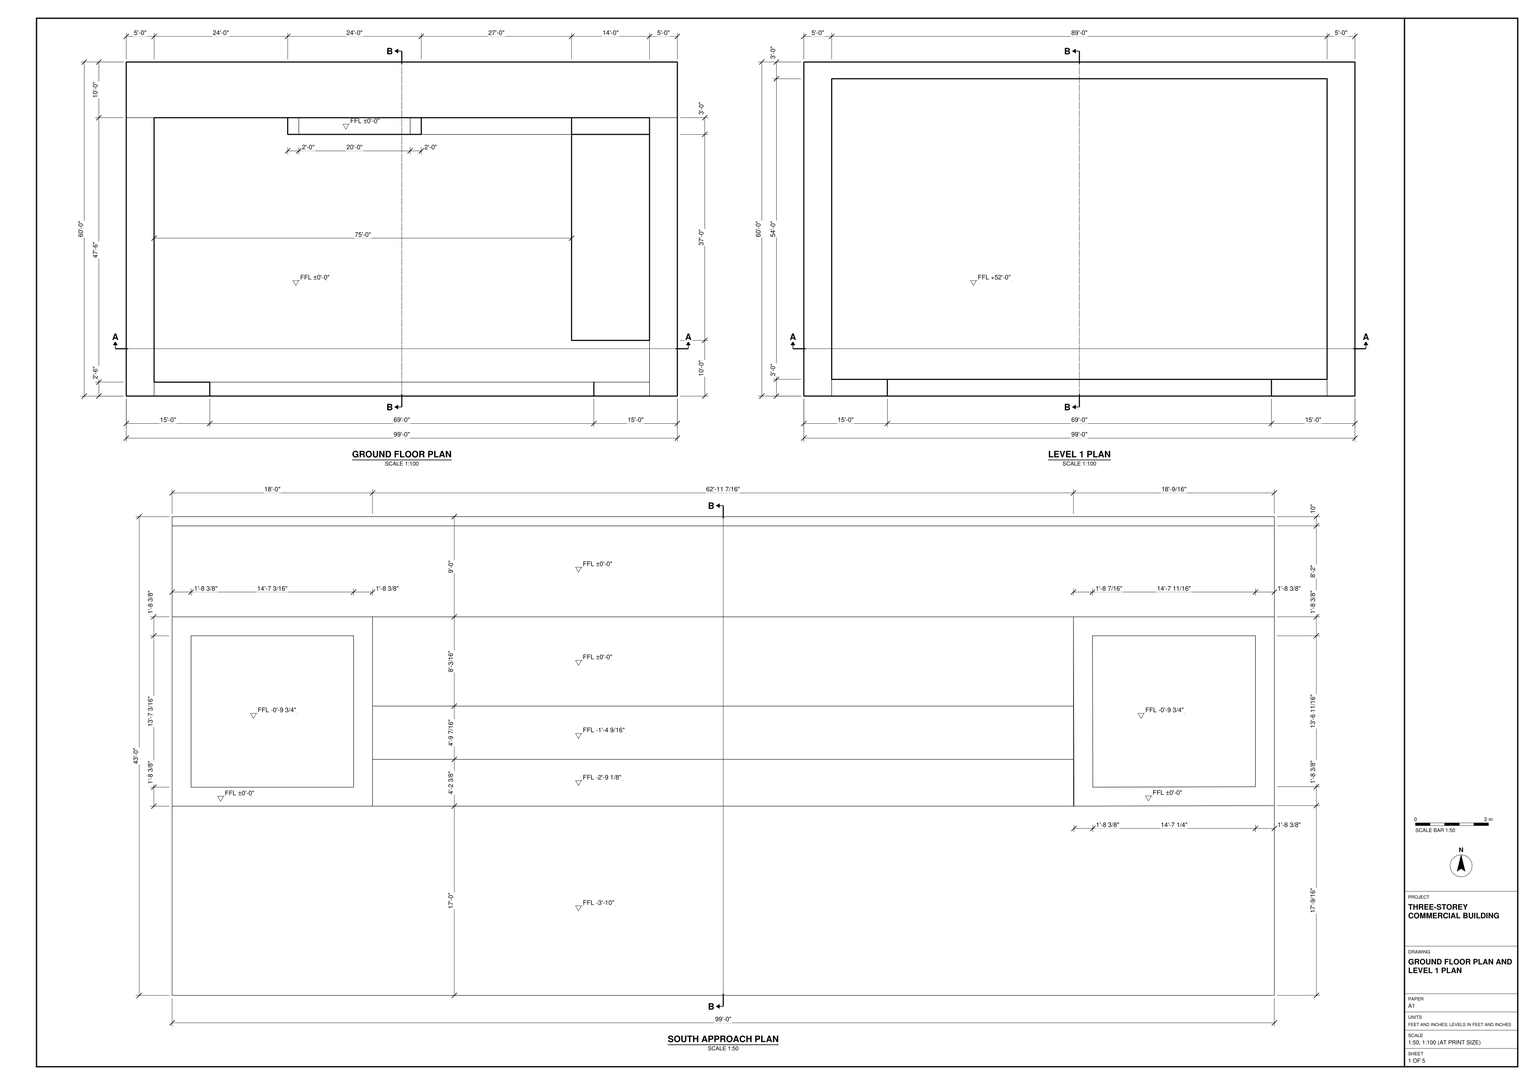
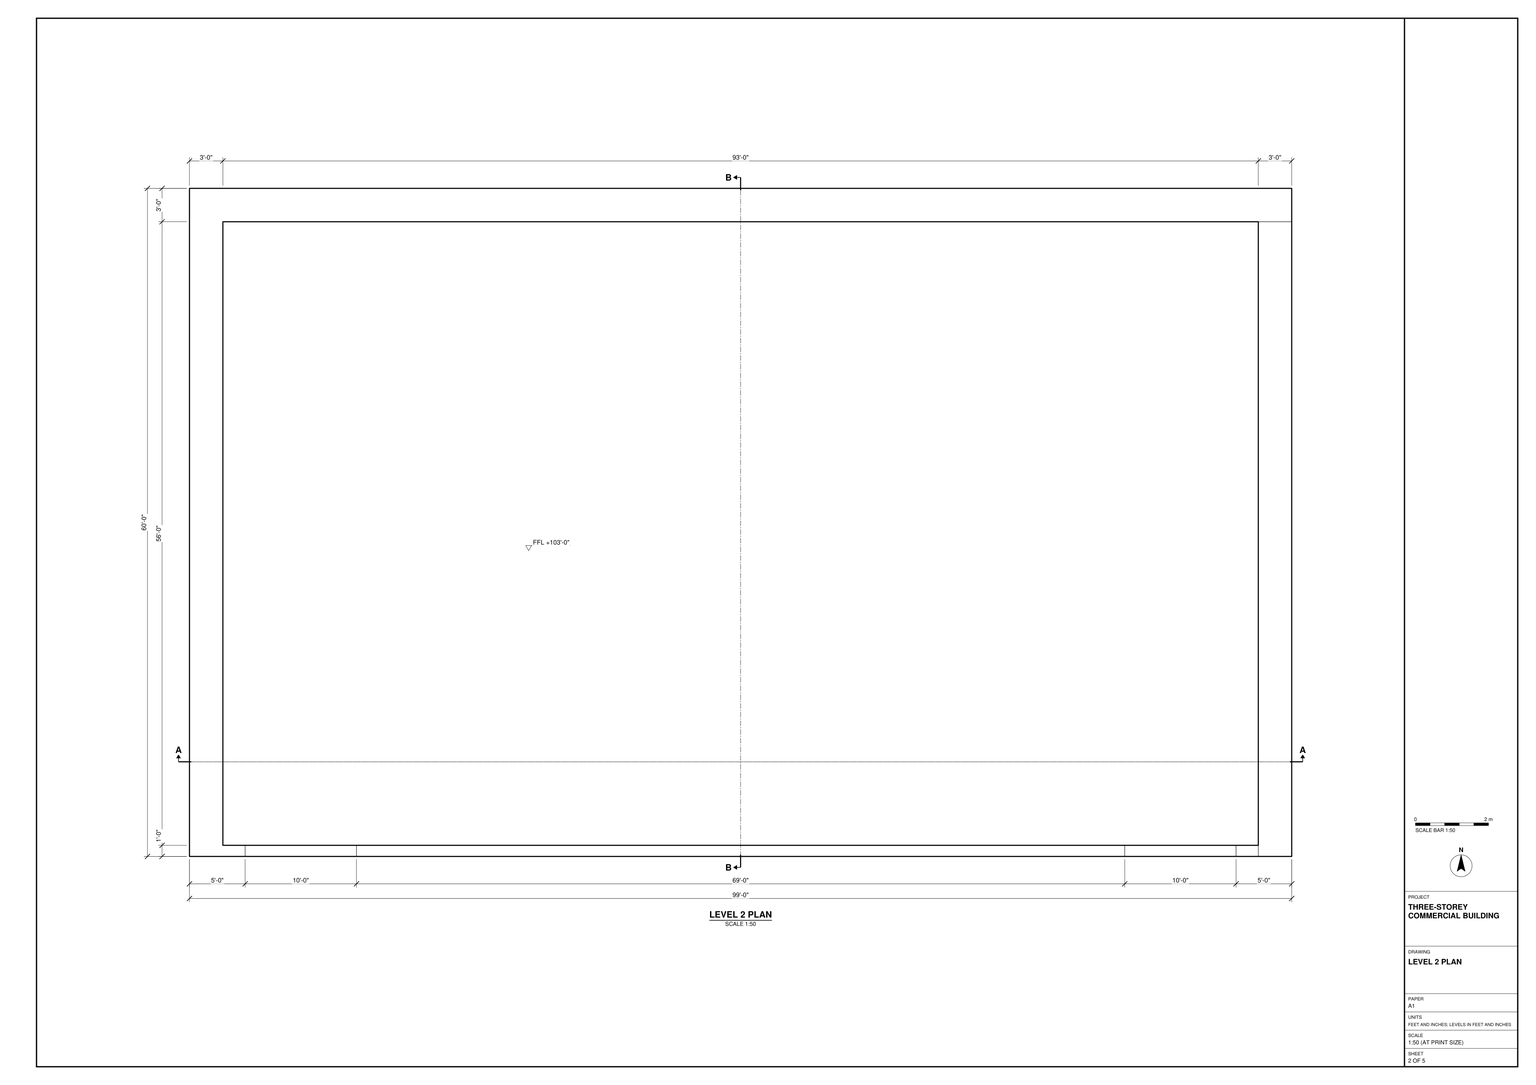
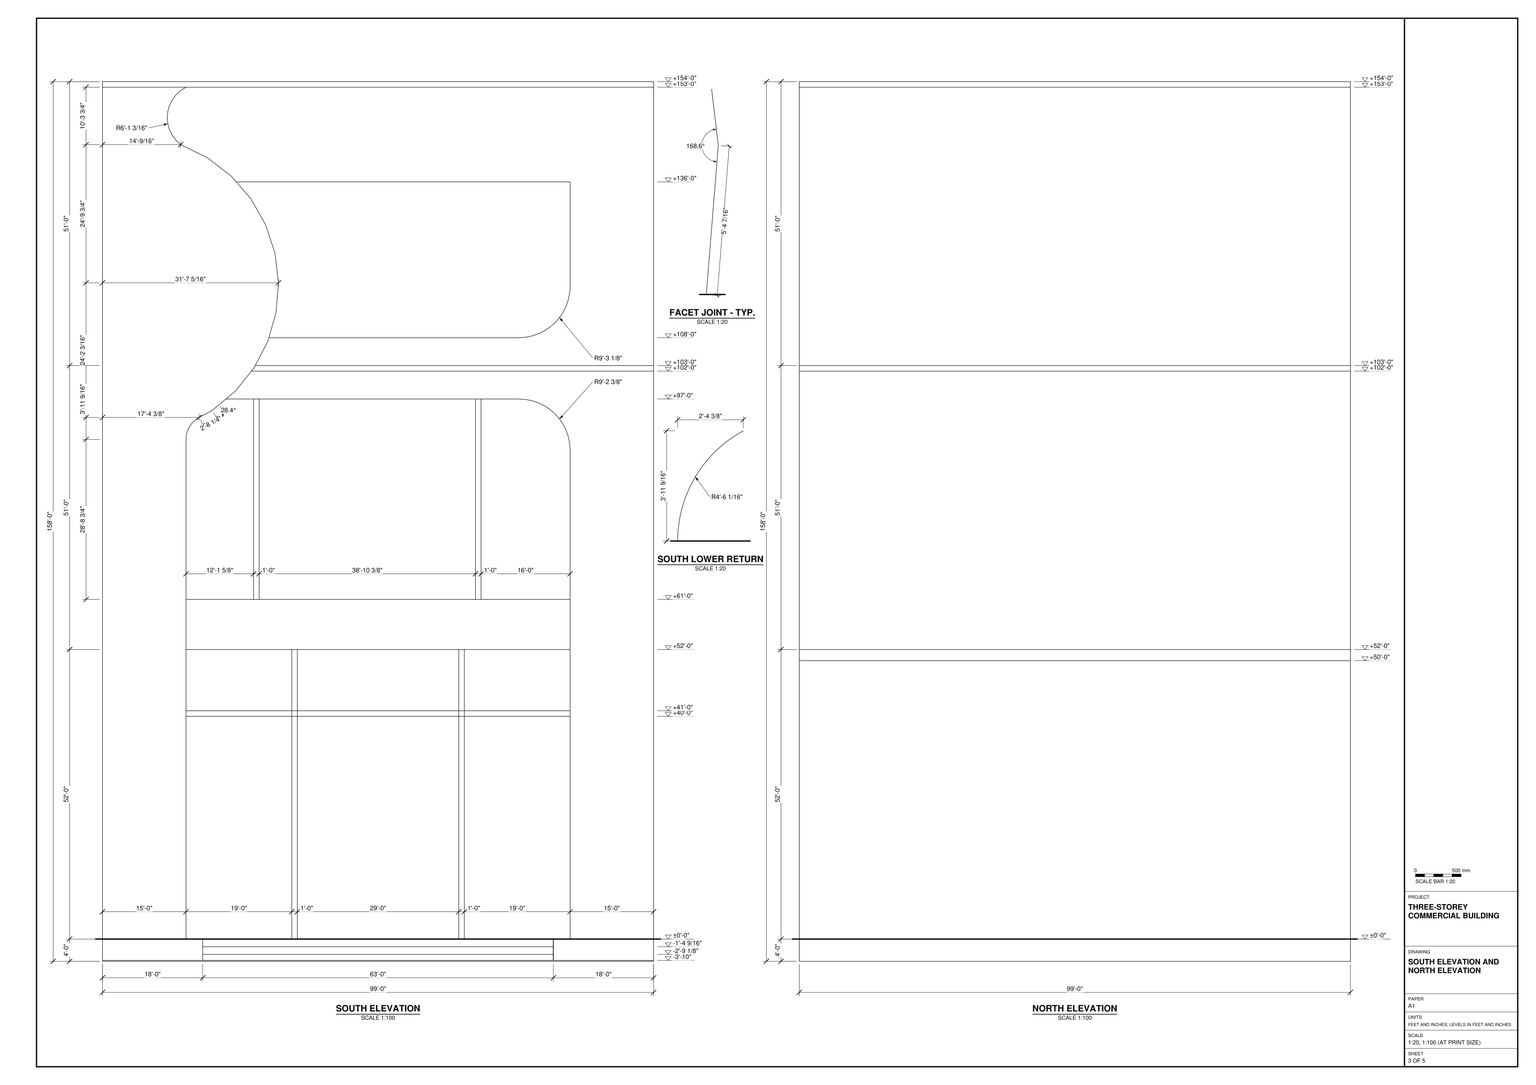
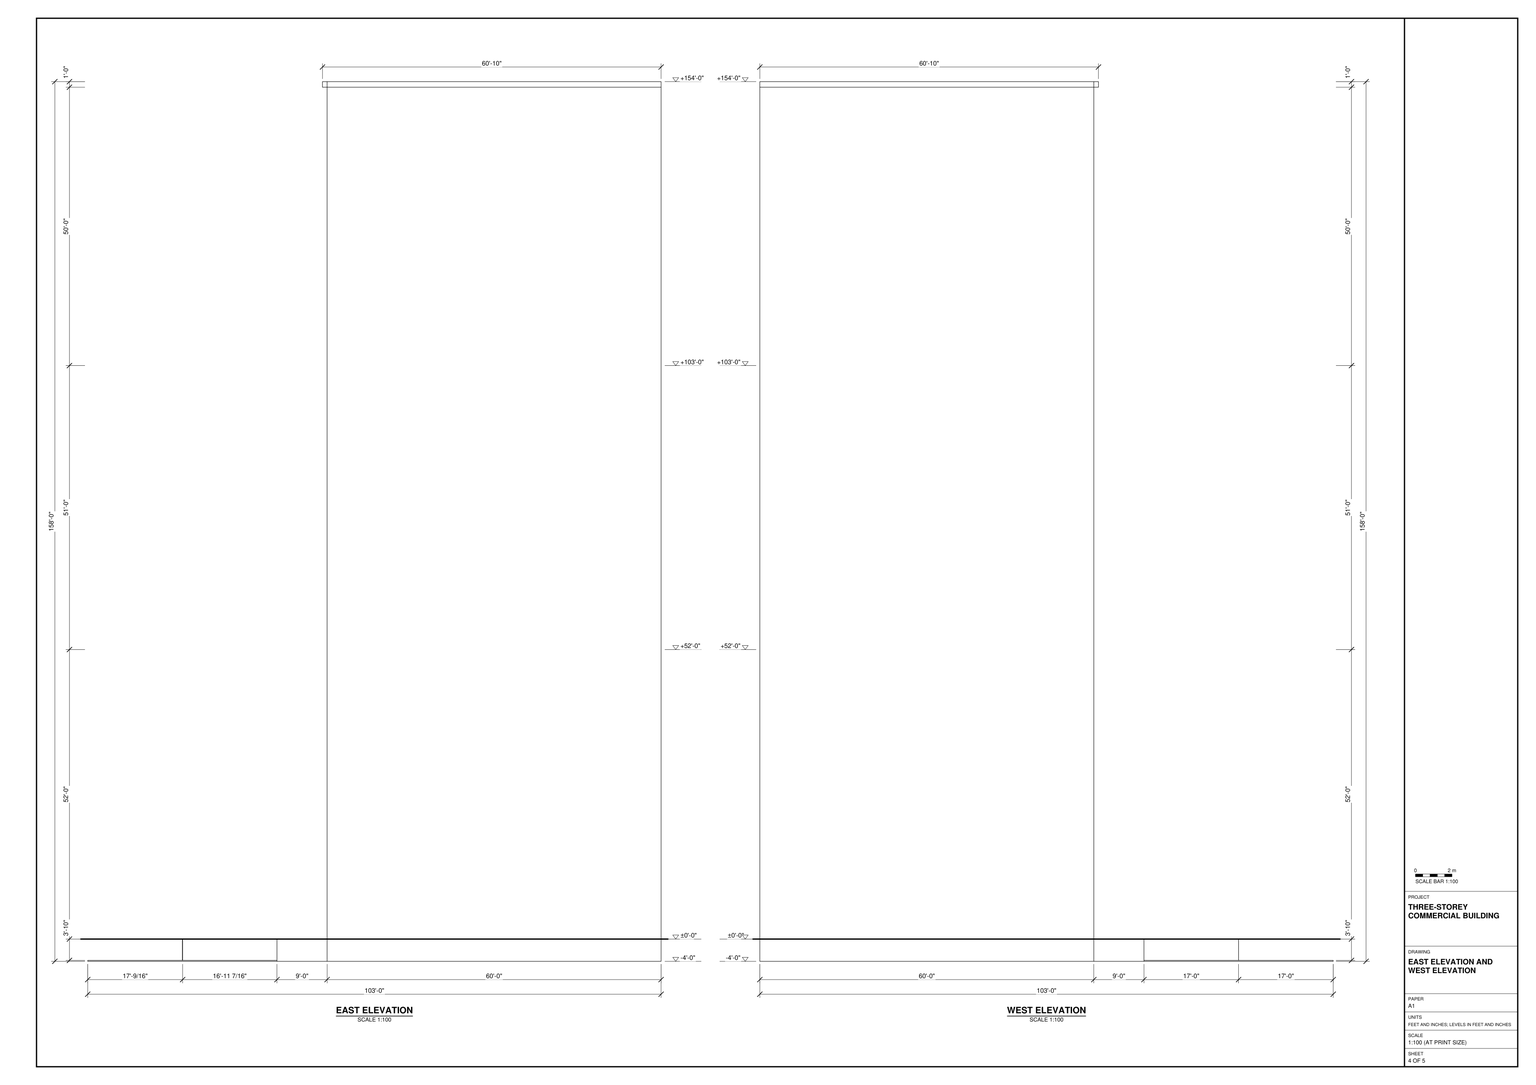
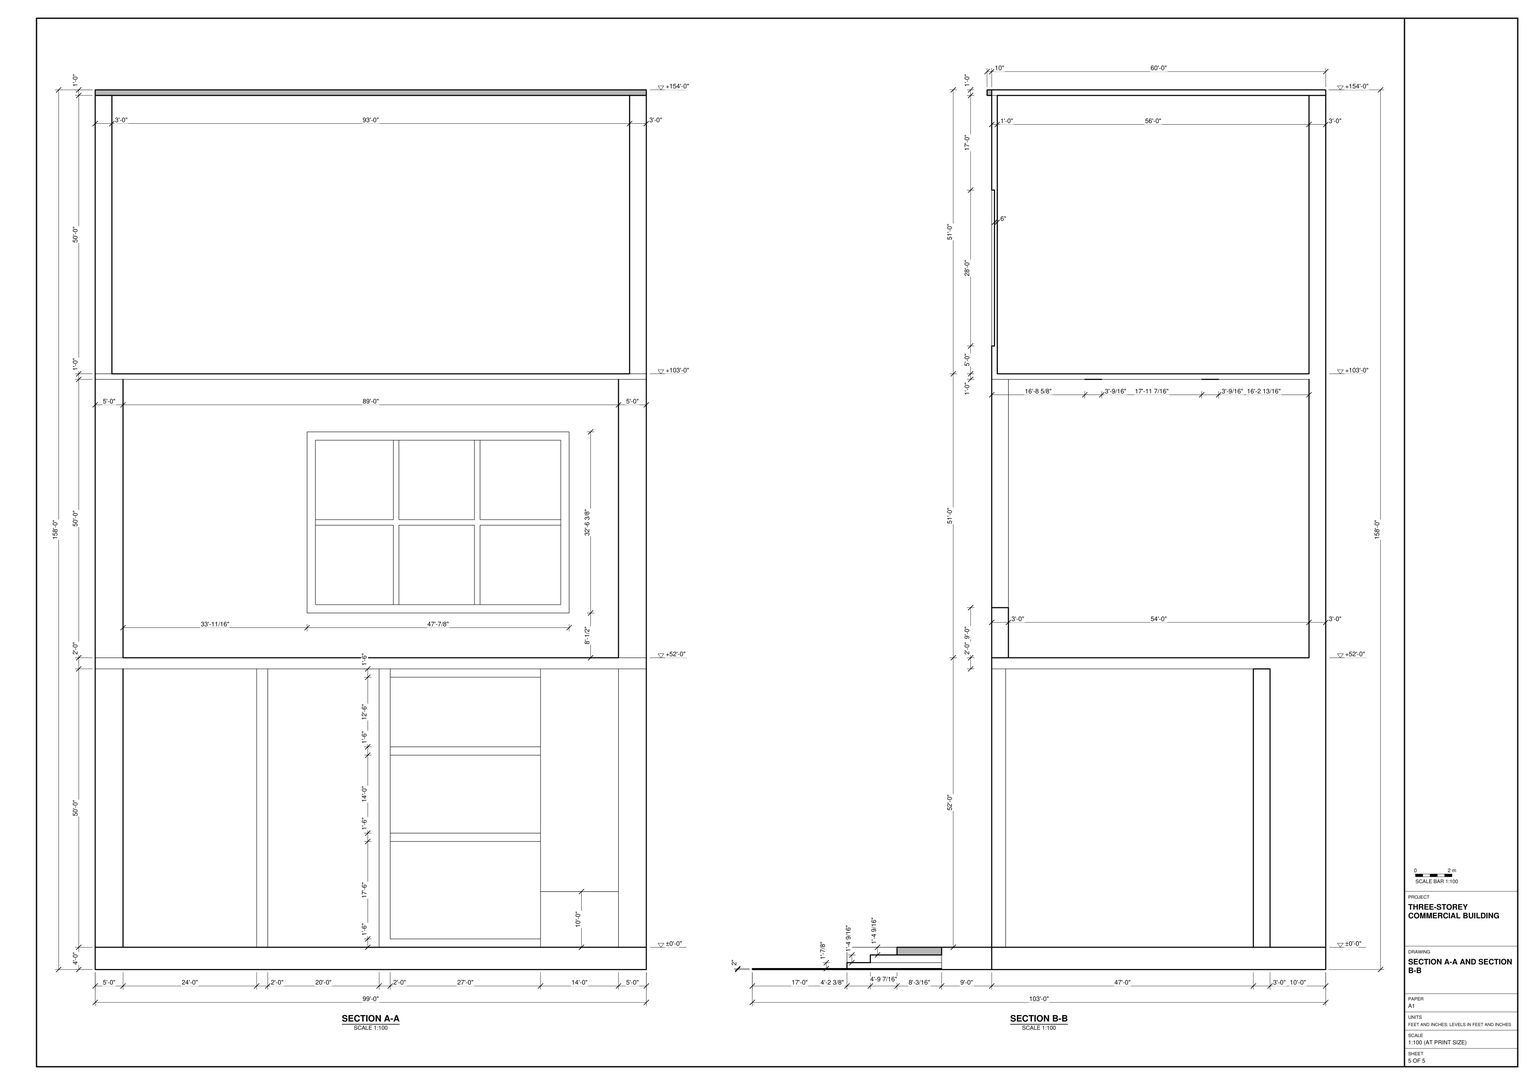
Build the three-storey commercial building and its south approach in SketchUp using task_files/diagram_01.pdf. Work in feet and inches. The complete model is 99'-0" wide from east to west, 103'-0" deep from north to south including the approach, and 158'-0" high from the underside of the base to the top of the roof. Set the floor levels at ±0'-0", +52'-0" and +103'-0".

Follow the plans for the wall thicknesses, wall returns and floor slab edges. Keep the upper floors open as drawn and cap the building with a flat roof slab. Use the south elevation to shape the front openings: follow the sweeping left edge across the upper storeys, round the indicated right-hand corners and place the framing divisions at the positions shown for each storey. Keep the north face plain apart from its horizontal slab lines. Extend the approach south of the building, with broad central steps leading up to the entrance landing and a bordered inset area on either side.

Keep walls, slabs, roof and approach elements separately grouped. Keep any furniture or joinery pieces shown as separate groups or components, and use components for repeated parts. Any decor or loose items shown may be suitable library components. Save one SketchUp model as output_files/three_storey_commercial_building_with_stepped_approach.skp.

# SketchUp Ruby script. Lengths in inches.
U = 1.inch
M = Sketchup.active_model
def pt(a) = Geom::Point3d.new(a.map { |v| v * U })
def face(e, loops, mat)
  f = e.add_face(loops[0].map { |a| pt(a) })
  loops[1..].each { |l| e.add_face(l.map { |a| pt(a) }).erase! }
  f.material = f.back_material = mat if mat
  f
end
# faces: each face lists its corners as indices into pts; further lists are holes
def faces(e, pts, list, mat = nil) = list.each { |f| face(e, (f[0].is_a?(Array) ? f : [f]).map { |l| l.map { |i| pts[i] } }, mat) }
# xy, xz, yz: faces in a plane at the given z, y or x. An outline is a flat list of corners, or four numbers for a rectangle; further outlines are holes
def ring(l) = l.size == 4 ? [[l[0], l[1]], [l[2], l[1]], [l[2], l[3]], [l[0], l[3]]] : l.each_slice(2).to_a
def flat(e, list, mat, &to3) = list.each { |f| face(e, (f[0].is_a?(Array) ? f : [f]).map { |l| ring(l).map { |u, v| to3.(u, v) } }, mat) }
def xy(e, z, list, mat = nil) = flat(e, list, mat) { |x, y| [x, y, z] }
def xz(e, y, list, mat = nil) = flat(e, list, mat) { |x, z| [x, y, z] }
def yz(e, x, list, mat = nil) = flat(e, list, mat) { |y, z| [x, y, z] }
def lines(e, pts, list) = list.each { |a, b| e.add_line(pt(pts[a]), pt(pts[b])) }
# prism: a flat outline (further loops are holes) pulled along v
def prism(e, loops, v, mat = nil)
  f = face(e, loops, mat); d = Geom::Vector3d.new(v.map { |x| x * U })
  f.pushpull(f.normal.samedirection?(d) ? d.length : -d.length)
end
def box(e, o, s, mat = nil) = prism(e, [[o, [o[0] + s[0], o[1], o[2]], [o[0] + s[0], o[1] + s[1], o[2]], [o[0], o[1] + s[1], o[2]]]], [0, 0, s[2]], mat)
def at(x, y, z, deg = 0) = Geom::Transformation.translation(pt([x, y, z])) * Geom::Transformation.rotation(ORIGIN, Z_AXIS, deg.degrees)
def axes(o, x, y, z) = Geom::Transformation.new([*x, 0, *y, 0, *z, 0, *pt(o).to_a, 1])
def part(name) = M.definitions.add(name)
# library, detail: a bought-in or finely detailed component or shape, given as its bounding box
def library(name, o, s) = part(name).tap { |d| box(d.entities, o, s) }
def detail(e, o, s) = box(e.add_group.entities, o, s)
def put(e, d, t, mat = nil) = e.add_instance(d, t).tap { |i| i.material = mat if mat }
def group(e, t, mat = nil) = e.add_group.tap { |g| g.transformation = t; g.material = mat if mat }.entities
root = M.entities
M.materials.add("[0011_Seashell]").color = [255, 245, 238]
M.materials.add("[0036_BurlyWood]").color = [178, 147, 108]
M.materials.add("[0111_SlateGray]").color = [37, 43, 48]
M.materials.add("[0136_Charcoal]").color = [35, 35, 35]
M.materials.add("[Granite Dark Gray]").color = [69, 68, 68]
M.materials.add("[Grass Dark Green]").color = [106, 157, 55]
M.materials.add("[Pavers with Grass Herringbone]").color = [102, 100, 96]
M.materials.add("[Stone Masonry Multi]").color = [182, 175, 164]
M.materials.add("[Stone Vein Gray]").color = [166, 165, 165]
M.materials.add("[Translucent Glass Gray]").color = [76, 76, 76]
M.materials["[Translucent Glass Gray]"].alpha = 0.5
M.materials.add("[Translucent Glass Gray]1").color = [173, 173, 173]
M.materials["[Translucent Glass Gray]1"].alpha = 0.5
M.materials.add("[Wood Cherry Original]").color = [152, 86, 42]
M.materials.add("[Wood Veneer 01]").color = [89, 52, 27]
M.materials.add("[Wood Veneer 01]1").color = [120, 70, 37]
xy(root,-36,[[0,0,1188,408],[0,408,1188,516],[0,516,1188,1236]])
xy(root,-34,[[[0,204,216,408],[20.4,224.4,195.6,387.6]],[216,204,971.45,408],[[972,204,971.45,408,1188,408,1188,204.58],[992.34,224.45,1167.6,224.93,1167.6,387.6,991.91,387.6]]])
xy(root,-34,[[0,0,1188,0,1188,204.58,972,204,971.45,408,971.45,204,0,204]],"[Pavers with Grass Herringbone]")
xy(root,-21.12,[[216,204,971.45,254.375]],"[Granite Dark Gray]")
xy(root,-4.56,[[216,311.8125,971.45,408]])
xy(root,-4.56,[[216,254.375,971.45,311.8125]],"[Granite Dark Gray]")
xy(root,2.25,[[20.4,224.4,195.6,387.6],[992.34,224.45,1167.6,224.93,1167.6,387.6,991.91,387.6]],"[Grass Dark Green]")
xy(root,12,[[0,516,60,1116],[60,516,180,546],[180,516,1008,546],[1008,516,1128,546],[1128,516,1188,1116],
  [960,636,1128,1080],[636,1080,636,1116,0,1116,0,1236,1188,1236,1188,1116,960,1116,960,1080],[348,1080,372,1116],[372,1080,612,1116],[612,1080,636,1116],
  [960,1080,1128,1116]])
xy(root,12,[[[0,204,216,408],[20.4,224.4,195.6,387.6]],[[972,204,1188,204.58,1188,408,971.45,408],[992.34,224.45,991.91,387.6,1167.6,387.6,1167.6,224.93]],[216,311.8125,971.45,408],[0,408,1188,516]],"[Granite Dark Gray]")
xy(root,12,[[60,546,1128,546,1128,636,960,636,960,1080,348,1080,348,1116,60,1116]],"[Stone Vein Gray]")
xy(root,30,[[636,1080,960,1116]],"[Wood Cherry Original]")
xy(root,132,[[960,636,1128,1080]],"[Wood Cherry Original]")
xy(root,240,[[636,1080,960,1116]],"[Wood Cherry Original]")
xy(root,258,[[636,1080,960,1116]],"[Wood Veneer 01]1")
xy(root,426,[[636,1080,960,1116]],"[Wood Cherry Original]")
xy(root,444,[[636,1080,960,1116]],"[Wood Cherry Original]")
xy(root,594,[[636,1080,960,1116]],"[Wood Cherry Original]")
xy(root,612,[[241.63,762.29,235.48,763.5,229.86,766.26,225.14,770.38,221.65,775.59,219.625,781.51,219.2,787.77,220.41,793.91,223.17,799.54,227.29,804.26,232.5,807.75,238.43,809.77,244.68,810.19,250.82,808.98,256.45,806.22,261.17,802.1,264.66,796.9,266.68,790.97,267.11,784.72,265.89,778.57,263.13,772.95,259.01,768.23,253.81,764.74,247.88,762.71],[505.63,762.29,499.48,763.5,493.86,766.26,489.14,770.38,485.65,775.59,483.625,781.51,483.2,787.77,484.41,793.91,487.17,799.54,491.29,804.26,496.5,807.75,502.43,809.77,508.68,810.19,514.82,808.98,520.45,806.22,525.17,802.1,528.66,796.9,530.68,790.97,531.11,784.72,529.89,778.57,527.13,772.95,523.01,768.23,517.81,764.74,511.88,762.71],[769.63,762.29,763.48,763.5,757.86,766.26,753.14,770.38,749.65,775.59,747.625,781.51,747.2,787.77,748.41,793.91,751.17,799.54,755.29,804.26,760.5,807.75,766.43,809.77,772.68,810.19,778.82,808.98,784.45,806.22,789.17,802.1,792.66,796.9,794.68,790.97,795.11,784.72,793.89,778.57,791.13,772.95,787.01,768.23,781.81,764.74,775.88,762.71],[1033.63,762.29,1027.48,763.5,1021.86,766.26,1017.14,770.38,1013.65,775.59,1011.625,781.51,1011.2,787.77,1012.41,793.91,1015.17,799.54,1019.29,804.26,1024.5,807.75,1030.43,809.77,1036.68,810.19,1042.82,808.98,1048.45,806.22,1053.17,802.1,1056.66,796.9,1058.68,790.97,1059.11,784.72,1057.89,778.57,1055.13,772.95,1051.01,768.23,1045.81,764.74,1039.88,762.71],[348,1080,636,1116],
  [348,1080,636,1116],[636,1080,960,1116],[960,1080,1128,1116]])
xy(root,636,[[180,516,1008,552]])
xy(root,636,[[60,552,1128,1200]],"[Stone Vein Gray]")
xy(root,744,[[180,516,1008,552]])
xy(root,1236,[[357.26,710.92,351.05,711.73,345.26,714.13,340.29,717.94,336.48,722.92,334.08,728.7,333.26,734.92,334.08,741.125,336.48,746.92,340.29,751.89,345.26,755.7,351.05,758.1,357.26,758.92,363.47,758.1,369.26,755.7,374.23,751.89,378.05,746.92,380.44,741.125,381.26,734.92,380.44,728.7,378.05,722.92,374.23,717.94,369.26,714.13,363.47,711.73],[609.26,710.92,603.05,711.73,597.26,714.13,592.29,717.94,588.48,722.92,586.08,728.7,585.26,734.92,586.08,741.125,588.48,746.92,592.29,751.89,597.26,755.7,603.05,758.1,609.26,758.92,615.47,758.1,621.26,755.7,626.23,751.89,630.05,746.92,632.44,741.125,633.26,734.92,632.44,728.7,630.05,722.92,626.23,717.94,621.26,714.13,615.47,711.73],[861.26,710.92,855.05,711.73,849.26,714.13,844.29,717.94,840.48,722.92,838.08,728.7,837.26,734.92,838.08,741.125,840.48,746.92,844.29,751.89,849.26,755.7,855.05,758.1,861.26,758.92,867.47,758.1,873.26,755.7,878.23,751.89,882.05,746.92,884.44,741.125,885.26,734.92,884.44,728.7,882.05,722.92,878.23,717.94,873.26,714.13,867.47,711.73],[357.26,962.92,351.05,963.73,345.26,966.13,340.29,969.94,336.48,974.92,334.08,980.7,333.26,986.92,334.08,993.125,336.48,998.92,340.29,1003.89,345.26,1007.7,351.05,1010.1,357.26,1010.92,363.47,1010.1,369.26,1007.7,374.23,1003.89,378.05,998.92,380.44,993.125,381.26,986.92,380.44,980.7,378.05,974.92,374.23,969.94,369.26,966.13,363.47,963.73],[609.26,962.92,603.05,963.73,597.26,966.13,592.29,969.94,588.48,974.92,586.08,980.7,585.26,986.92,586.08,993.125,588.48,998.92,592.29,1003.89,597.26,1007.7,603.05,1010.1,609.26,1010.92,615.47,1010.1,621.26,1007.7,626.23,1003.89,630.05,998.92,632.44,993.125,633.26,986.92,632.44,980.7,630.05,974.92,626.23,969.94,621.26,966.13,615.47,963.73],
  [861.26,962.92,855.05,963.73,849.26,966.13,844.29,969.94,840.48,974.92,838.08,980.7,837.26,986.92,838.08,993.125,840.48,998.92,844.29,1003.89,849.26,1007.7,855.05,1010.1,861.26,1010.92,867.47,1010.1,873.26,1007.7,878.23,1003.89,882.05,998.92,884.44,993.125,885.26,986.92,884.44,980.7,882.05,974.92,878.23,969.94,873.26,966.13,867.47,963.73]])
xy(root,1248,[[36,528,1152,1200]],"[Wood Cherry Original]")
xy(root,1308,[[358.54,516,896.89,522]])
xy(root,1644,[[288.26,516,1008,522]])
xy(root,1848,[[0,506,36,516],[36,506,180,516],[180,506,1152,516],[1152,506,1188,516],[0,516,0,1236,1188,1236,1188,1200,36,1200,36,516],
  [1152,516,1188,1200],[36,528,1152,1200]])
xy(root,1860,[[0,506,1188,516],[0,516,1188,1236]])
xz(root,0,[[0,-36,1188,-34]])
xz(root,204,[[0,-34,216,12],[216,-34,971.45,-21.12]],"[Granite Dark Gray]")
xz(root,224.4,[[20.4,2.25,195.6,12]])
xz(root,224.4,[[20.4,-34,195.6,2.25]],"[Grass Dark Green]")
xz(root,254.375,[[216,-21.12,971.45,-4.56]],"[Granite Dark Gray]")
xz(root,311.8125,[[216,-4.56,971.45,12]],"[Granite Dark Gray]")
xz(root,387.6,[[20.4,2.25,195.6,12],[991.91,2.25,1167.6,12]],"[Granite Dark Gray]")
xz(root,387.6,[[20.4,-34,195.6,2.25],[991.91,-34,1167.6,2.25]],"[Grass Dark Green]")
xz(root,408,[[0,-36,1188,-34],[0,-34,216,12],[971.45,-34,1188,12],[216,-4.56,971.45,12]])
xz(root,506,[[0,1848,1188,1860]])
xz(root,516,[[0,-36,1188,12],[0,1848,1188,1860]])
xz(root,516,[[180,636,1008,744]],"[0111_SlateGray]")
xz(root,516,[[408,12,420,492],[768,12,780,492],[180,492,408,504],[408,492,420,504],[420,492,768,504],
  [768,492,780,504],[780,492,1008,504],[408,504,420,636],[768,504,780,636],[325.625,744,337.625,1176],
  [804,744,816,1176],[320.96,1236,1188,1236,1188,1248,329.21,1248,326.65,1243.08]],"[0136_Charcoal]")
xz(root,516,[[0,12,180,12,180,1088.75,180.22,1093.59,180.87,1098.39,181.94,1103.11,183.4375,1107.71,185.34,1112.17,187.63,1116.43,190.29,1120.47,193.31,1124.26,196.65,1127.77,200.29,1130.96,204.2,1133.81,208.36,1136.3,236.71,1151.62,266,1176,286.25,1192.86,320.96,1236,326.65,1243.08,329.21,1248,356.33,1300.3,358.54,1308,374.12,1362.25,379.3,1426.5,371.68,1490.51,351.5625,1551.74,319.73,1607.79,288.26,1644,277.45,1656.45,226.38,1695.78,168.55,1724.24,158.6,1733.33,150.49,1744.1,144.49,1756.17,140.8,1769.14,139.5625,1782.5625,140.8,1795.99,144.49,1808.95,150.49,1821.02,158.6,1831.79,168.55,1840.89,180,1848,0,1848]],"[Stone Masonry Multi]")
xz(root,516,[[180,12,408,492],[420,12,768,492],[780,12,1008,492],[180,504,408,636],[420,504,768,636],
  [780,504,1008,636],[180,744,325.625,744,325.625,1176,266,1176,236.71,1151.62,208.36,1136.3,204.2,1133.81,200.29,1130.96,196.65,1127.77,193.31,1124.26,190.29,1120.47,187.63,1116.43,185.34,1112.17,183.4375,1107.71,181.94,1103.11,180.87,1098.39,180.22,1093.59,180,1088.75],[337.625,744,804,1176],[816,744,1008,744,1008,1065.64,1007.06,1080.05,1004.24,1094.21,999.6,1107.875,993.21,1120.82,985.19,1132.82,975.68,1143.68,964.82,1153.19,952.82,1161.21,939.875,1167.6,926.21,1172.24,912.05,1175.06,897.64,1176,816,1176]],"[Translucent Glass Gray]")
xz(root,516,[[1008,12,1188,12,1188,1236,320.96,1236,286.25,1192.86,266,1176,897.64,1176,912.05,1175.06,926.21,1172.24,939.875,1167.6,952.82,1161.21,964.82,1153.19,975.68,1143.68,985.19,1132.82,993.21,1120.82,999.6,1107.875,1004.24,1094.21,1007.06,1080.05,1008,1065.64],[329.21,1248,1188,1248,1188,1848,180,1848,168.55,1840.89,158.6,1831.79,150.49,1821.02,144.49,1808.95,140.8,1795.99,139.5625,1782.5625,140.8,1769.14,144.49,1756.17,150.49,1744.1,158.6,1733.33,168.55,1724.24,226.38,1695.78,277.45,1656.45,288.26,1644,1008,1644,1008,1419.11,1007.05,1404.61,1004.21,1390.36,999.54,1376.59,993.11,1363.56,985.04,1351.47,975.46,1340.54,964.53,1330.96,952.44,1322.89,939.41,1316.46,925.64,1311.79,911.39,1308.95,896.89,1308,358.54,1308,356.33,1300.3]],"[Wood Cherry Original]")
xz(root,522,[[358.54,1308,896.89,1308,911.39,1308.95,925.64,1311.79,939.41,1316.46,952.44,1322.89,964.53,1330.96,975.46,1340.54,985.04,1351.47,993.11,1363.56,999.54,1376.59,1004.21,1390.36,1007.05,1404.61,1008,1419.11,1008,1644,288.26,1644,319.73,1607.79,351.5625,1551.74,371.68,1490.51,379.3,1426.5,374.12,1362.25]],"[Translucent Glass Gray]1")
xz(root,528,[[36,1248,1152,1848]])
xz(root,546,[[60,12,180,612]])
xz(root,552,[[60,636,180,1236],[180,636,1008,744],[1008,636,1128,1236]])
xz(root,636,[[960,12,1128,132]],"[Wood Cherry Original]")
xz(root,1080,[[960,12,1128,132]])
xz(root,1080,[[372,12,612,612],[960,132,1128,612],[636,426,960,444],[636,594,960,612]],"[Wood Cherry Original]")
xz(root,1080,[[348,12,372,612],[612,12,960,12,960,30,636,30,636,612,612,612],[636,240,960,258]],"[Wood Veneer 01]")
xz(root,1116,[[348,12,372,612],[372,12,612,612],[612,12,636,612],[960,12,1128,612],[636,594,960,612]])
xz(root,1116,[[60,12,348,612],[636,30,960,240],[636,258,960,426],[636,444,960,594]],"[Wood Cherry Original]")
xz(root,1200,[[36,1248,1152,1848]])
xz(root,1200,[[[60,636,1128,1236],[456.71,732.47,1021.59,1122.85]]],"[0036_BurlyWood]")
xz(root,1200,[[[456.71,732.47,1021.59,1122.85],[474.71,750.47,1003.59,1104.85]],[642.71,750.47,654.71,750.47,654.71,921.66,817.59,921.66,817.59,750.47,829.59,750.47,829.59,921.66,1003.59,921.66,1003.59,933.66,829.59,933.66,829.59,1104.85,817.59,1104.85,817.59,933.66,654.71,933.66,654.71,1104.85,642.71,1104.85,642.71,933.66,474.71,933.66,474.71,921.66,642.71,921.66]],"[0136_Charcoal]")
xz(root,1200,[[474.71,750.47,642.71,921.66],[654.71,750.47,817.59,921.66],[829.59,750.47,1003.59,921.66],[474.71,933.66,642.71,1104.85],[654.71,933.66,817.59,1104.85],
  [829.59,933.66,1003.59,1104.85]],"[Translucent Glass Gray]")
xz(root,1236,[[0,612,1188,636],[0,1236,1188,1248],[0,1848,1188,1860]])
xz(root,1236,[[0,-36,1188,12],[0,12,1188,612],[0,636,1188,1236],[0,1248,1188,1848]],"[0011_Seashell]")
yz(root,0,[[0,-36,408,-34],[506,1848,516,1860],[516,1848,1236,1860]])
yz(root,0,[[516,-36,1236,12],[516,12,1236,1848]],"[0011_Seashell]")
yz(root,0,[[408,-36,516,12],[204,-34,408,12]],"[Granite Dark Gray]")
yz(root,20.4,[[224.4,2.25,387.6,12]],"[Granite Dark Gray]")
yz(root,20.4,[[224.4,-34,387.6,2.25]],"[Grass Dark Green]")
yz(root,36,[[528,1248,1200,1848]])
yz(root,60,[[552,636,1200,1236]],"[0036_BurlyWood]")
yz(root,60,[[546,12,1116,612]],"[Wood Veneer 01]1")
yz(root,180,[[516,12,546,612],[516,636,552,744]])
yz(root,195.6,[[224.4,2.25,387.6,12]],"[Granite Dark Gray]")
yz(root,195.6,[[224.4,-34,387.6,2.25]],"[Grass Dark Green]")
yz(root,216,[[204,-34,408,-21.12],[254.375,-21.12,408,-4.56],[311.8125,-4.56,408,12]])
yz(root,216,[[204,-21.12,254.375,-21.12,254.375,-4.56,311.8125,-4.56,311.8125,12,204,12]],"[Granite Dark Gray]")
yz(root,348,[[1080,12,1116,612]],"[Wood Cherry Original]")
yz(root,636,[[1080,240,1116,258],[1080,426,1116,444],[1080,594,1116,612]])
yz(root,636,[[1080,30,1116,240],[1080,258,1116,426],[1080,444,1116,594]],"[Wood Cherry Original]")
yz(root,960,[[1080,240,1116,258],[1080,426,1116,444],[1080,594,1116,612]])
yz(root,960,[[1080,258,1116,426],[1080,444,1116,594]],"[Wood Cherry Original]")
yz(root,960,[[[636,12,1080,132],[645,21,1071,123]],[645,21,1071,123],[1080,30,1116,240]],"[Wood Veneer 01]1")
yz(root,971.45,[[204,-34,408,-21.12],[254.375,-21.12,408,-4.56],[311.8125,-4.56,408,12]])
yz(root,1008,[[516,12,546,612],[516,636,552,744],[516,1419.11,522,1644]])
yz(root,1128,[[636,12,1080,132],[1080,12,1116,612]])
yz(root,1128,[[552,636,1200,1236]],"[0036_BurlyWood]")
yz(root,1152,[[528,1248,1200,1848]])
yz(root,1167.6,[[224.93,2.25,387.6,12]],"[Granite Dark Gray]")
yz(root,1167.6,[[224.93,-34,387.6,2.25]],"[Grass Dark Green]")
yz(root,1188,[[0,-36,408,-34],[506,1848,516,1860],[516,1848,1236,1860]])
yz(root,1188,[[516,-36,1236,12],[516,12,1236,1848]],"[0011_Seashell]")
yz(root,1188,[[408,-36,516,12],[204.58,-34,408,12]],"[Granite Dark Gray]")
p = [[971.45,408,-34],[972,204,-34],[972,204,12],[971.45,408,12],[971.45,408,-4.56],[971.45,408,-21.12],
  [1188,204.58,-34],[1188,204.58,12],[992.34,224.45,-34],[991.91,387.6,-34],[991.91,387.6,2.25],[992.34,224.45,2.25],
  [1167.6,224.93,-34],[1167.6,224.93,2.25],[992.34,224.45,12],[991.91,387.6,12],[1167.6,224.93,12],[374.12,516,1362.25],
  [358.54,516,1308],[358.54,522,1308],[374.12,522,1362.25],[896.89,516,1308],[911.39,516,1308.95],[911.39,522,1308.95],
  [896.89,522,1308],[925.64,516,1311.79],[925.64,522,1311.79],[939.41,516,1316.46],[939.41,522,1316.46],[952.44,516,1322.89],
  [952.44,522,1322.89],[964.53,516,1330.96],[964.53,522,1330.96],[975.46,516,1340.54],[975.46,522,1340.54],[985.04,516,1351.47],
  [985.04,522,1351.47],[993.11,516,1363.56],[993.11,522,1363.56],[379.3,516,1426.5],[379.3,522,1426.5],[999.54,516,1376.59],
  [999.54,522,1376.59],[1004.21,516,1390.36],[1004.21,522,1390.36],[1007.05,516,1404.61],[1007.05,522,1404.61],[1008,516,1419.11],
  [1008,522,1419.11],[371.68,516,1490.51],[371.68,522,1490.51],[351.5625,516,1551.74],[351.5625,522,1551.74],[319.73,516,1607.79],
  [319.73,522,1607.79],[288.26,516,1644],[288.26,522,1644],[1188,1116,612],[1128,1116,612],[1188,1080,612],
  [1128,1080,612],[60,516,636],[60,552,636],[60,516,1236],[60,552,1236],[1188,1200,1236],
  [1128,1200,1236],[1128,552,636],[1128,516,636],[60,546,612],[60,516,612],[1152,528,1248],
  [1152,516,1248],[1008,552,1236],[1008,516,1236],[1128,552,1236],[1128,516,1236],[180,552,1236],
  [180,516,1236]]
faces(root,p,[[0,1,2,3,4,5],[1,6,7,2],[14,11,10,15]],"[Granite Dark Gray]")
faces(root,p,[[8,9,10,11],[12,8,11,13]],"[Grass Dark Green]")
faces(root,p,[[16,13,11,14],[17,18,19,20],[21,22,23,24],[22,25,26,23],[25,27,28,26],[27,29,30,28],[29,31,32,30],[31,33,34,32],
  [33,35,36,34],[35,37,38,36],[39,17,20,40],[37,41,42,38],[41,43,44,42],[43,45,46,44],[45,47,48,46],[49,39,40,50],
  [51,49,50,52],[53,51,52,54],[55,53,54,56]])
lines(root,p,[[57,58],[59,60],[61,62],[63,64],[65,66],[67,68],[69,70],[71,72],[73,74],[75,76],[77,78]])
